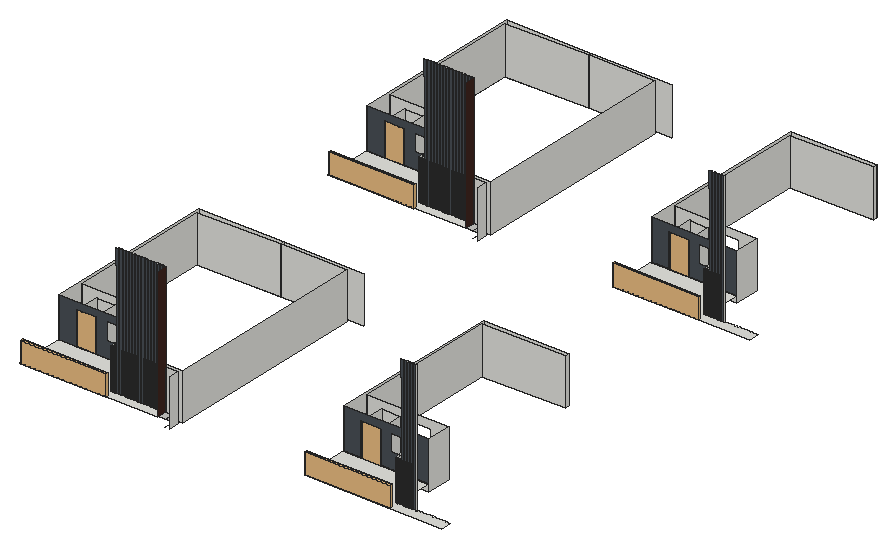
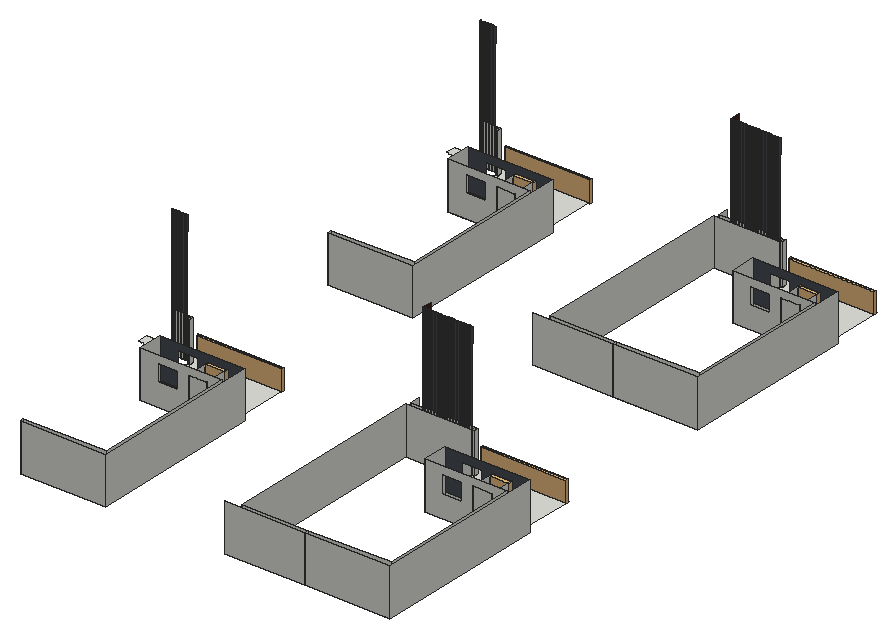
# SketchUp Ruby script. Lengths in inches.
U = 1.inch
M = Sketchup.active_model
def pt(a) = Geom::Point3d.new(a.map { |v| v * U })
def face(e, loops, mat)
  f = e.add_face(loops[0].map { |a| pt(a) })
  loops[1..].each { |l| e.add_face(l.map { |a| pt(a) }).erase! }
  f.material = f.back_material = mat if mat
  f
end
# faces: each face lists its corners as indices into pts; further lists are holes
def faces(e, pts, list, mat = nil) = list.each { |f| face(e, (f[0].is_a?(Array) ? f : [f]).map { |l| l.map { |i| pts[i] } }, mat) }
# xy, xz, yz: faces in a plane at the given z, y or x. An outline is a flat list of corners, or four numbers for a rectangle; further outlines are holes
def ring(l) = l.size == 4 ? [[l[0], l[1]], [l[2], l[1]], [l[2], l[3]], [l[0], l[3]]] : l.each_slice(2).to_a
def flat(e, list, mat, &to3) = list.each { |f| face(e, (f[0].is_a?(Array) ? f : [f]).map { |l| ring(l).map { |u, v| to3.(u, v) } }, mat) }
def xy(e, z, list, mat = nil) = flat(e, list, mat) { |x, y| [x, y, z] }
def xz(e, y, list, mat = nil) = flat(e, list, mat) { |x, z| [x, y, z] }
def yz(e, x, list, mat = nil) = flat(e, list, mat) { |y, z| [x, y, z] }
def lines(e, pts, list) = list.each { |a, b| e.add_line(pt(pts[a]), pt(pts[b])) }
# prism: a flat outline (further loops are holes) pulled along v
def prism(e, loops, v, mat = nil)
  f = face(e, loops, mat); d = Geom::Vector3d.new(v.map { |x| x * U })
  f.pushpull(f.normal.samedirection?(d) ? d.length : -d.length)
end
def box(e, o, s, mat = nil) = prism(e, [[o, [o[0] + s[0], o[1], o[2]], [o[0] + s[0], o[1] + s[1], o[2]], [o[0], o[1] + s[1], o[2]]]], [0, 0, s[2]], mat)
def at(x, y, z, deg = 0) = Geom::Transformation.translation(pt([x, y, z])) * Geom::Transformation.rotation(ORIGIN, Z_AXIS, deg.degrees)
def axes(o, x, y, z) = Geom::Transformation.new([*x, 0, *y, 0, *z, 0, *pt(o).to_a, 1])
def part(name) = M.definitions.add(name)
# library, detail: a bought-in or finely detailed component or shape, given as its bounding box
def library(name, o, s) = part(name).tap { |d| box(d.entities, o, s) }
def detail(e, o, s) = box(e.add_group.entities, o, s)
def put(e, d, t, mat = nil) = e.add_instance(d, t).tap { |i| i.material = mat if mat }
def group(e, t, mat = nil) = e.add_group.tap { |g| g.transformation = t; g.material = mat if mat }.entities
root = M.entities
M.materials.add("[0043_SaddleBrown]").color = [63, 38, 31]
M.materials.add("[Formica Blue]").color = [73, 80, 86]
c1 = library("door (1)",[38.93,25.48,0],[40,9.94,82.68])
c2 = library("Glass Railing",[0,0,0],[139.5,4.76,42])
xy(root,384.25,[[348.1875,438.72,353.97,447.84],[1072.625,438.72,1078.41,447.84],[137.5,535.375,137.5,980.35,353.97,980.35,353.97,971.23,144.84,965.96,144.84,540.48,353.97,540.48,353.97,535.375],[861.9375,535.375,861.9375,980.35,1078.41,980.35,1078.41,971.23,869.28,965.96,869.28,540.48,1078.41,540.48,1078.41,535.375],[144.84,540.48,353.97,598.8125],
  [869.28,540.48,1078.41,598.8125],[348.1875,1419.07,353.97,1428.19],[1072.625,1419.07,1078.41,1428.19],[137.5,1515.73,137.5,1960.7,353.97,1960.7,353.97,1951.58,144.84,1946.3125,144.84,1520.83,353.97,1520.83,353.97,1515.73],[861.9375,1515.73,861.9375,1960.7,1078.41,1960.7,1078.41,1951.58,869.28,1946.3125,869.28,1520.83,1078.41,1520.83,1078.41,1515.73],
  [144.84,1520.83,353.97,1579.16],[869.28,1520.83,1078.41,1579.16]])
xy(root,401.6875,[[137.5,412.04,487.0625,412.04,487.0625,437.1,481.3,437.1,481.3,438.72,479.0625,438.72,479.0625,437.1,473.3,437.1,473.3,438.72,471.0625,438.72,471.0625,437.1,465.3,437.1,465.3,438.72,463.0625,438.72,463.0625,437.1,457.3,437.1,457.3,438.72,455.0625,438.72,455.0625,437.1,449.3,437.1,449.3,438.72,447.0625,438.72,447.0625,437.1,441.3,437.1,441.3,438.72,439.0625,438.72,439.0625,437.1,433.3,437.1,433.3,438.72,431.0625,438.72,431.0625,437.1,425.3,437.1,425.3,438.72,423.0625,438.72,423.0625,437.1,417.3,437.1,417.3,438.72,415.0625,438.72,415.0625,437.1,409.3,437.1,409.3,438.72,407.0625,438.72,407.0625,437.1,401.3,437.1,401.3,438.72,399.0625,438.72,399.0625,437.1,393.3,437.1,393.3,438.72,391.0625,438.72,391.0625,437.1,385.3,437.1,385.3,438.72,383.0625,438.72,383.0625,437.1,377.3,437.1,377.3,438.72,375.0625,438.72,375.0625,437.1,369.3,437.1,369.3,438.72,367.0625,438.72,367.0625,437.1,361.3,437.1,361.3,438.72,358.875,438.72,358.875,437.1,353.97,437.1,353.97,438.72,352.41,438.72,352.41,437.1,348.1875,437.1,348.1875,447.84,353.97,447.84,353.97,535.375,137.5,535.375],[861.9375,412.04,1211.5,412.04,1211.5,437.1,1205.74,437.1,1205.74,438.72,1203.5,438.72,1203.5,437.1,1197.74,437.1,1197.74,438.72,1195.5,438.72,1195.5,437.1,1189.74,437.1,1189.74,438.72,1187.5,438.72,1187.5,437.1,1181.74,437.1,1181.74,438.72,1179.5,438.72,1179.5,437.1,1173.74,437.1,1173.74,438.72,1171.5,438.72,1171.5,437.1,1165.74,437.1,1165.74,438.72,1163.5,438.72,1163.5,437.1,1157.74,437.1,1157.74,438.72,1155.5,438.72,1155.5,437.1,1149.74,437.1,1149.74,438.72,1147.5,438.72,1147.5,437.1,1141.74,437.1,1141.74,438.72,1139.5,438.72,1139.5,437.1,1133.74,437.1,1133.74,438.72,1131.5,438.72,1131.5,437.1,1125.74,437.1,1125.74,438.72,1123.5,438.72,1123.5,437.1,1117.74,437.1,1117.74,438.72,1115.5,438.72,1115.5,437.1,1109.74,437.1,1109.74,438.72,1107.5,438.72,1107.5,437.1,1101.74,437.1,1101.74,438.72,1099.5,438.72,1099.5,437.1,1093.74,437.1,1093.74,438.72,1091.5,438.72,1091.5,437.1,1085.74,437.1,1085.74,438.72,1083.3125,438.72,1083.3125,437.1,1078.41,437.1,1078.41,438.72,1076.85,438.72,1076.85,437.1,1072.625,437.1,1072.625,447.84,1078.41,447.84,1078.41,535.375,861.9375,535.375],[348.1875,437.1,352.41,438.72],[353.97,437.1,358.875,438.72],[361.3,437.1,367.0625,438.72],
  [369.3,437.1,375.0625,438.72],[377.3,437.1,383.0625,438.72],[385.3,437.1,391.0625,438.72],[393.3,437.1,399.0625,438.72],[401.3,437.1,407.0625,438.72],
  [409.3,437.1,415.0625,438.72],[417.3,437.1,423.0625,438.72],[425.3,437.1,431.0625,438.72],[433.3,437.1,439.0625,438.72],[441.3,437.1,447.0625,438.72],
  [449.3,437.1,455.0625,438.72],[457.3,437.1,463.0625,438.72],[465.3,437.1,471.0625,438.72],[473.3,437.1,479.0625,438.72],[481.3,437.1,487.0625,438.72],
  [1072.625,437.1,1076.85,438.72],[1078.41,437.1,1083.3125,438.72],[1085.74,437.1,1091.5,438.72],[1093.74,437.1,1099.5,438.72],[1101.74,437.1,1107.5,438.72],
  [1109.74,437.1,1115.5,438.72],[1117.74,437.1,1123.5,438.72],[1125.74,437.1,1131.5,438.72],[183.3,535.375,231.3,598.8125],[907.74,535.375,955.74,598.8125],
  [137.5,1392.39,487.0625,1392.39,487.0625,1417.45,481.3,1417.45,481.3,1419.07,479.0625,1419.07,479.0625,1417.45,473.3,1417.45,473.3,1419.07,471.0625,1419.07,471.0625,1417.45,465.3,1417.45,465.3,1419.07,463.0625,1419.07,463.0625,1417.45,457.3,1417.45,457.3,1419.07,455.0625,1419.07,455.0625,1417.45,449.3,1417.45,449.3,1419.07,447.0625,1419.07,447.0625,1417.45,441.3,1417.45,441.3,1419.07,439.0625,1419.07,439.0625,1417.45,433.3,1417.45,433.3,1419.07,431.0625,1419.07,431.0625,1417.45,425.3,1417.45,425.3,1419.07,423.0625,1419.07,423.0625,1417.45,417.3,1417.45,417.3,1419.07,415.0625,1419.07,415.0625,1417.45,409.3,1417.45,409.3,1419.07,407.0625,1419.07,407.0625,1417.45,401.3,1417.45,401.3,1419.07,399.0625,1419.07,399.0625,1417.45,393.3,1417.45,393.3,1419.07,391.0625,1419.07,391.0625,1417.45,385.3,1417.45,385.3,1419.07,383.0625,1419.07,383.0625,1417.45,377.3,1417.45,377.3,1419.07,375.0625,1419.07,375.0625,1417.45,369.3,1417.45,369.3,1419.07,367.0625,1419.07,367.0625,1417.45,361.3,1417.45,361.3,1419.07,358.875,1419.07,358.875,1417.45,353.97,1417.45,353.97,1419.07,352.41,1419.07,352.41,1417.45,348.1875,1417.45,348.1875,1428.19,353.97,1428.19,353.97,1515.73,137.5,1515.73],[861.9375,1392.39,1211.5,1392.39,1211.5,1417.45,1205.74,1417.45,1205.74,1419.07,1203.5,1419.07,1203.5,1417.45,1197.74,1417.45,1197.74,1419.07,1195.5,1419.07,1195.5,1417.45,1189.74,1417.45,1189.74,1419.07,1187.5,1419.07,1187.5,1417.45,1181.74,1417.45,1181.74,1419.07,1179.5,1419.07,1179.5,1417.45,1173.74,1417.45,1173.74,1419.07,1171.5,1419.07,1171.5,1417.45,1165.74,1417.45,1165.74,1419.07,1163.5,1419.07,1163.5,1417.45,1157.74,1417.45,1157.74,1419.07,1155.5,1419.07,1155.5,1417.45,1149.74,1417.45,1149.74,1419.07,1147.5,1419.07,1147.5,1417.45,1141.74,1417.45,1141.74,1419.07,1139.5,1419.07,1139.5,1417.45,1133.74,1417.45,1133.74,1419.07,1131.5,1419.07,1131.5,1417.45,1125.74,1417.45,1125.74,1419.07,1123.5,1419.07,1123.5,1417.45,1117.74,1417.45,1117.74,1419.07,1115.5,1419.07,1115.5,1417.45,1109.74,1417.45,1109.74,1419.07,1107.5,1419.07,1107.5,1417.45,1101.74,1417.45,1101.74,1419.07,1099.5,1419.07,1099.5,1417.45,1093.74,1417.45,1093.74,1419.07,1091.5,1419.07,1091.5,1417.45,1085.74,1417.45,1085.74,1419.07,1083.3125,1419.07,1083.3125,1417.45,1078.41,1417.45,1078.41,1419.07,1076.85,1419.07,1076.85,1417.45,1072.625,1417.45,1072.625,1428.19,1078.41,1428.19,1078.41,1515.73,861.9375,1515.73],[348.1875,1417.45,352.41,1419.07],[353.97,1417.45,358.875,1419.07],[361.3,1417.45,367.0625,1419.07],
  [369.3,1417.45,375.0625,1419.07],[377.3,1417.45,383.0625,1419.07],[385.3,1417.45,391.0625,1419.07],[393.3,1417.45,399.0625,1419.07],[401.3,1417.45,407.0625,1419.07],
  [409.3,1417.45,415.0625,1419.07],[417.3,1417.45,423.0625,1419.07],[425.3,1417.45,431.0625,1419.07],[433.3,1417.45,439.0625,1419.07],[441.3,1417.45,447.0625,1419.07],
  [449.3,1417.45,455.0625,1419.07],[457.3,1417.45,463.0625,1419.07],[465.3,1417.45,471.0625,1419.07],[473.3,1417.45,479.0625,1419.07],[481.3,1417.45,487.0625,1419.07],
  [1072.625,1417.45,1076.85,1419.07],[1078.41,1417.45,1083.3125,1419.07],[1085.74,1417.45,1091.5,1419.07],[1093.74,1417.45,1099.5,1419.07],[1101.74,1417.45,1107.5,1419.07],
  [1109.74,1417.45,1115.5,1419.07],[1117.74,1417.45,1123.5,1419.07],[183.3,1515.73,231.3,1579.16],[907.74,1515.73,955.74,1579.16]])
xz(root,437.1,[[348.1875,401.6875,352.41,504.25],[353.97,401.6875,358.875,504.25],[361.3,401.6875,367.0625,401.6875,367.0625,733.125,361.3,733.125,361.3,693.65,363.73,693.65,363.73,504.25,361.3,504.25],[369.3,401.6875,375.0625,733.125],[377.3,401.6875,383.0625,733.125],
  [385.3,401.6875,391.0625,733.125],[393.3,401.6875,399.0625,733.125],[401.3,401.6875,407.0625,733.125],[409.3,401.6875,415.0625,733.125],[417.3,401.6875,423.0625,733.125],
  [425.3,401.6875,431.0625,733.125],[433.3,401.6875,439.0625,733.125],[441.3,401.6875,447.0625,733.125],[449.3,401.6875,455.0625,733.125],[457.3,401.6875,463.0625,733.125],
  [465.3,401.6875,471.0625,733.125],[473.3,401.6875,479.0625,733.125],[481.3,401.6875,487.0625,733.125],[1072.625,401.6875,1076.85,504.25],[1078.41,401.6875,1083.3125,504.25],
  [1085.74,401.6875,1091.5,401.6875,1091.5,733.125,1085.74,733.125,1085.74,693.65,1088.17,693.65,1088.17,504.25,1085.74,504.25],[1093.74,401.6875,1099.5,733.125],[1101.74,401.6875,1107.5,733.125],[1109.74,401.6875,1115.5,733.125],[1117.74,401.6875,1123.5,733.125]],"[Formica Blue]")
xz(root,438.72,[[348.1875,384.25,353.97,401.6875],[353.97,384.25,504.5,401.6875],[1072.625,384.25,1078.41,401.6875]])
xz(root,438.72,[[352.41,401.6875,353.97,504.25],[358.875,401.6875,361.3,504.25],[367.0625,401.6875,369.3,733.125],[375.0625,401.6875,377.3,733.125],[383.0625,401.6875,385.3,733.125],
  [391.0625,401.6875,393.3,733.125],[399.0625,401.6875,401.3,733.125],[407.0625,401.6875,409.3,733.125],[415.0625,401.6875,417.3,733.125],[423.0625,401.6875,425.3,733.125],
  [431.0625,401.6875,433.3,733.125],[439.0625,401.6875,441.3,733.125],[447.0625,401.6875,449.3,733.125],[455.0625,401.6875,457.3,733.125],[463.0625,401.6875,465.3,733.125],
  [471.0625,401.6875,473.3,733.125],[479.0625,401.6875,481.3,733.125],[1076.85,401.6875,1078.41,504.25],[1083.3125,401.6875,1085.74,504.25],[1091.5,401.6875,1093.74,733.125],
  [1099.5,401.6875,1101.74,733.125],[1107.5,401.6875,1109.74,733.125],[1115.5,401.6875,1117.74,733.125],[1123.5,401.6875,1125.74,733.125]],"[Formica Blue]")
xz(root,447.84,[[348.1875,384.25,353.97,401.6875],[353.97,384.25,521.63,504.25],[1072.625,384.25,1078.41,401.6875],[348.1875,401.6875,353.97,504.25],[1072.625,401.6875,1078.41,504.25]])
xz(root,535.375,[[137.5,384.25,353.97,401.6875],[861.9375,384.25,1078.41,401.6875]])
xz(root,535.375,[[[137.5,401.6875,183.3,401.6875,183.3,485.6875,231.3,485.6875,231.3,401.6875,353.97,401.6875,353.97,504.25,137.5,504.25],[258.09,441.5,309.84,485.6875]],[[861.9375,401.6875,907.74,401.6875,907.74,485.6875,955.74,485.6875,955.74,401.6875,1078.41,401.6875,1078.41,504.25,861.9375,504.25],[982.53,441.5,1034.28,485.6875]]],"[Formica Blue]")
xz(root,598.8125,[[[144.84,384.25,353.97,504.25],[183.3,401.6875,231.3,485.6875],[258.09,441.5,309.84,485.6875]],[[869.28,384.25,1078.41,504.25],[907.74,401.6875,955.74,485.6875],[982.53,441.5,1034.28,485.6875]],[183.3,401.6875,231.3,485.6875],[907.74,401.6875,955.74,485.6875]])
xz(root,971.23,[[353.97,384.25,521.63,504.25]])
xz(root,980.35,[[137.5,384.25,353.97,504.25],[353.97,384.25,558.625,504.25],[861.9375,384.25,1078.41,504.25]])
xz(root,1417.45,[[348.1875,401.6875,352.41,504.25],[353.97,401.6875,358.875,504.25],[361.3,401.6875,367.0625,401.6875,367.0625,733.125,361.3,733.125,361.3,693.65,363.73,693.65,363.73,504.25,361.3,504.25],[369.3,401.6875,375.0625,733.125],[377.3,401.6875,383.0625,733.125],
  [385.3,401.6875,391.0625,733.125],[393.3,401.6875,399.0625,733.125],[401.3,401.6875,407.0625,733.125],[409.3,401.6875,415.0625,733.125],[417.3,401.6875,423.0625,733.125],
  [425.3,401.6875,431.0625,733.125],[433.3,401.6875,439.0625,733.125],[441.3,401.6875,447.0625,733.125],[449.3,401.6875,455.0625,733.125],[457.3,401.6875,463.0625,733.125],
  [465.3,401.6875,471.0625,733.125],[473.3,401.6875,479.0625,733.125],[481.3,401.6875,487.0625,733.125],[1072.625,401.6875,1076.85,504.25],[1078.41,401.6875,1083.3125,504.25],
  [1085.74,401.6875,1091.5,401.6875,1091.5,733.125,1085.74,733.125,1085.74,693.65,1088.17,693.65,1088.17,504.25,1085.74,504.25],[1093.74,401.6875,1099.5,733.125],[1101.74,401.6875,1107.5,733.125],[1109.74,401.6875,1115.5,733.125],[1117.74,401.6875,1123.5,733.125]],"[Formica Blue]")
xz(root,1419.07,[[348.1875,384.25,353.97,401.6875],[353.97,384.25,504.5,401.6875],[1072.625,384.25,1078.41,401.6875]])
xz(root,1419.07,[[352.41,401.6875,353.97,504.25],[358.875,401.6875,361.3,504.25],[367.0625,401.6875,369.3,733.125],[375.0625,401.6875,377.3,733.125],[383.0625,401.6875,385.3,733.125],
  [391.0625,401.6875,393.3,733.125],[399.0625,401.6875,401.3,733.125],[407.0625,401.6875,409.3,733.125],[415.0625,401.6875,417.3,733.125],[423.0625,401.6875,425.3,733.125],
  [431.0625,401.6875,433.3,733.125],[439.0625,401.6875,441.3,733.125],[447.0625,401.6875,449.3,733.125],[455.0625,401.6875,457.3,733.125],[463.0625,401.6875,465.3,733.125],
  [471.0625,401.6875,473.3,733.125],[479.0625,401.6875,481.3,733.125],[1076.85,401.6875,1078.41,504.25],[1083.3125,401.6875,1085.74,504.25],[1091.5,401.6875,1093.74,733.125],
  [1099.5,401.6875,1101.74,733.125],[1107.5,401.6875,1109.74,733.125],[1115.5,401.6875,1117.74,733.125],[1123.5,401.6875,1125.74,733.125]],"[Formica Blue]")
xz(root,1428.19,[[348.1875,384.25,353.97,401.6875],[353.97,384.25,521.63,504.25],[1072.625,384.25,1078.41,401.6875],[348.1875,401.6875,353.97,504.25],[1072.625,401.6875,1078.41,504.25]])
xz(root,1515.73,[[137.5,384.25,353.97,401.6875],[861.9375,384.25,1078.41,401.6875]])
xz(root,1515.73,[[[137.5,401.6875,183.3,401.6875,183.3,485.6875,231.3,485.6875,231.3,401.6875,353.97,401.6875,353.97,504.25,137.5,504.25],[258.09,441.5,309.84,485.6875]],[[861.9375,401.6875,907.74,401.6875,907.74,485.6875,955.74,485.6875,955.74,401.6875,1078.41,401.6875,1078.41,504.25,861.9375,504.25],[982.53,441.5,1034.28,485.6875]]],"[Formica Blue]")
xz(root,1579.16,[[[144.84,384.25,353.97,504.25],[183.3,401.6875,231.3,485.6875],[258.09,441.5,309.84,485.6875]],[[869.28,384.25,1078.41,504.25],[907.74,401.6875,955.74,485.6875],[982.53,441.5,1034.28,485.6875]],[183.3,401.6875,231.3,485.6875],[907.74,401.6875,955.74,485.6875]])
xz(root,1951.58,[[353.97,384.25,521.63,504.25]])
xz(root,1960.7,[[137.5,384.25,353.97,504.25],[353.97,384.25,558.625,504.25],[861.9375,384.25,1078.41,504.25]])
yz(root,137.5,[[535.375,384.25,980.35,504.25],[1515.73,384.25,1960.7,504.25]])
yz(root,144.84,[[598.8125,384.25,965.96,504.25],[1579.16,384.25,1946.3125,504.25]])
yz(root,183.3,[[535.375,401.6875,598.8125,485.6875],[1515.73,401.6875,1579.16,485.6875]])
yz(root,231.3,[[535.375,401.6875,598.8125,485.6875],[1515.73,401.6875,1579.16,485.6875]])
yz(root,348.1875,[[438.72,384.25,447.84,401.6875],[1419.07,384.25,1428.19,401.6875],[437.1,401.6875,447.84,504.25],[1417.45,401.6875,1428.19,504.25]])
yz(root,352.41,[[437.1,401.6875,438.72,504.25],[1417.45,401.6875,1419.07,504.25]])
yz(root,353.97,[[438.72,384.25,447.84,504.25],[535.375,384.25,598.8125,504.25],[971.23,384.25,980.35,504.25],[1419.07,384.25,1428.19,504.25],[1515.73,384.25,1579.16,504.25],
  [1951.58,384.25,1960.7,504.25],[437.1,401.6875,438.72,504.25],[1417.45,401.6875,1419.07,504.25]])
yz(root,358.875,[[437.1,401.6875,438.72,504.25],[1417.45,401.6875,1419.07,504.25]])
yz(root,361.3,[[437.1,401.6875,438.72,504.25],[1417.45,401.6875,1419.07,504.25]])
yz(root,367.0625,[[437.1,401.6875,438.72,504.25],[1417.45,401.6875,1419.07,504.25]])
yz(root,369.3,[[437.1,401.6875,438.72,733.125],[1417.45,401.6875,1419.07,733.125]])
yz(root,375.0625,[[437.1,401.6875,438.72,504.25],[1417.45,401.6875,1419.07,504.25]])
yz(root,377.3,[[437.1,401.6875,438.72,733.125],[1417.45,401.6875,1419.07,733.125]])
yz(root,383.0625,[[437.1,401.6875,438.72,504.25],[1417.45,401.6875,1419.07,504.25]])
yz(root,385.3,[[437.1,401.6875,438.72,733.125],[1417.45,401.6875,1419.07,733.125]])
yz(root,391.0625,[[437.1,401.6875,438.72,504.25],[1417.45,401.6875,1419.07,504.25]])
yz(root,393.3,[[437.1,401.6875,438.72,733.125],[1417.45,401.6875,1419.07,733.125]])
yz(root,399.0625,[[437.1,401.6875,438.72,504.25],[1417.45,401.6875,1419.07,504.25]])
yz(root,401.3,[[437.1,401.6875,438.72,733.125],[1417.45,401.6875,1419.07,733.125]])
yz(root,407.0625,[[437.1,401.6875,438.72,504.25],[1417.45,401.6875,1419.07,504.25]])
yz(root,409.3,[[437.1,401.6875,438.72,733.125],[1417.45,401.6875,1419.07,733.125]])
yz(root,415.0625,[[437.1,401.6875,438.72,504.25],[1417.45,401.6875,1419.07,504.25]])
yz(root,417.3,[[437.1,401.6875,438.72,733.125],[1417.45,401.6875,1419.07,733.125]])
yz(root,423.0625,[[437.1,401.6875,438.72,504.25],[1417.45,401.6875,1419.07,504.25]])
yz(root,425.3,[[437.1,401.6875,438.72,733.125],[1417.45,401.6875,1419.07,733.125]])
yz(root,431.0625,[[437.1,401.6875,438.72,504.25],[1417.45,401.6875,1419.07,504.25]])
yz(root,433.3,[[437.1,401.6875,438.72,733.125],[1417.45,401.6875,1419.07,733.125]])
yz(root,439.0625,[[437.1,401.6875,438.72,504.25],[1417.45,401.6875,1419.07,504.25]])
yz(root,441.3,[[437.1,401.6875,438.72,733.125],[1417.45,401.6875,1419.07,733.125]])
yz(root,447.0625,[[437.1,401.6875,438.72,504.25],[1417.45,401.6875,1419.07,504.25]])
yz(root,449.3,[[437.1,401.6875,438.72,733.125],[1417.45,401.6875,1419.07,733.125]])
yz(root,455.0625,[[437.1,401.6875,438.72,504.25],[1417.45,401.6875,1419.07,504.25]])
yz(root,457.3,[[437.1,401.6875,438.72,733.125],[1417.45,401.6875,1419.07,733.125]])
yz(root,463.0625,[[437.1,401.6875,438.72,504.25],[1417.45,401.6875,1419.07,504.25]])
yz(root,465.3,[[437.1,401.6875,438.72,733.125],[1417.45,401.6875,1419.07,733.125]])
yz(root,471.0625,[[437.1,401.6875,438.72,504.25],[1417.45,401.6875,1419.07,504.25]])
yz(root,473.3,[[437.1,401.6875,438.72,733.125],[1417.45,401.6875,1419.07,733.125]])
yz(root,479.0625,[[437.1,401.6875,438.72,504.25],[1417.45,401.6875,1419.07,504.25]])
yz(root,481.3,[[437.1,401.6875,438.72,733.125],[1417.45,401.6875,1419.07,733.125]])
yz(root,487.0625,[[437.1,401.6875,438.72,504.25],[1417.45,401.6875,1419.07,504.25]])
yz(root,487.0625,[[412.04,401.6875,437.1,733.125],[1392.39,401.6875,1417.45,733.125]],"[0043_SaddleBrown]")
yz(root,517.3125,[[412.04,384.25,438.72,384.25,438.73,409.48,438.72,412.48,438.72,504.25,412.04,504.25],[1392.39,384.25,1419.07,384.25,1419.08,409.48,1419.07,412.48,1419.07,504.25,1392.39,504.25]])
yz(root,521.63,[[447.84,384.25,971.23,504.25],[1428.19,384.25,1951.58,504.25]])
yz(root,861.9375,[[535.375,384.25,980.35,504.25],[1515.73,384.25,1960.7,504.25]])
yz(root,869.28,[[598.8125,384.25,965.96,504.25],[1579.16,384.25,1946.3125,504.25]])
yz(root,907.74,[[535.375,401.6875,598.8125,485.6875],[1515.73,401.6875,1579.16,485.6875]])
yz(root,955.74,[[535.375,401.6875,598.8125,485.6875],[1515.73,401.6875,1579.16,485.6875]])
yz(root,1072.625,[[438.72,384.25,447.84,401.6875],[1419.07,384.25,1428.19,401.6875],[437.1,401.6875,447.84,504.25],[1417.45,401.6875,1428.19,504.25]])
yz(root,1076.85,[[437.1,401.6875,438.72,504.25],[1417.45,401.6875,1419.07,504.25]])
yz(root,1078.41,[[438.72,384.25,447.84,504.25],[535.375,384.25,598.8125,504.25],[971.23,384.25,980.35,504.25],[1419.07,384.25,1428.19,504.25],[1515.73,384.25,1579.16,504.25],
  [1951.58,384.25,1960.7,504.25],[437.1,401.6875,438.72,504.25],[1417.45,401.6875,1419.07,504.25]])
yz(root,1083.3125,[[437.1,401.6875,438.72,504.25],[1417.45,401.6875,1419.07,504.25]])
yz(root,1085.74,[[437.1,401.6875,438.72,504.25],[1417.45,401.6875,1419.07,504.25]])
yz(root,1091.5,[[437.1,401.6875,438.72,504.25],[1417.45,401.6875,1419.07,504.25]])
yz(root,1093.74,[[437.1,401.6875,438.72,733.125],[1417.45,401.6875,1419.07,733.125]])
yz(root,1099.5,[[437.1,401.6875,438.72,504.25],[1417.45,401.6875,1419.07,504.25]])
yz(root,1101.74,[[437.1,401.6875,438.72,733.125],[1417.45,401.6875,1419.07,733.125]])
yz(root,1107.5,[[437.1,401.6875,438.72,504.25],[1417.45,401.6875,1419.07,504.25]])
yz(root,1109.74,[[437.1,401.6875,438.72,733.125],[1417.45,401.6875,1419.07,733.125]])
yz(root,1115.5,[[437.1,401.6875,438.72,504.25],[1417.45,401.6875,1419.07,504.25]])
yz(root,1117.74,[[437.1,401.6875,438.72,733.125],[1417.45,401.6875,1419.07,733.125]])
yz(root,1123.5,[[437.1,401.6875,438.72,504.25],[1417.45,401.6875,1419.07,504.25]])
yz(root,1125.74,[[437.1,401.6875,438.72,733.125],[1417.45,401.6875,1419.07,733.125]])
p = [[504.5,438.72,384.25],[517.3125,438.72,384.25],[517.3125,438.73,409.48],[517.3125,438.72,412.48],[517.3125,438.72,504.25],[487.0625,438.72,504.25],
  [487.0625,438.72,401.6875],[504.5,438.72,401.6875],[144.84,965.96,384.25],[353.97,971.23,384.25],[353.97,971.23,504.25],[144.84,965.96,504.25],
  [869.28,965.96,384.25],[1078.41,971.23,384.25],[1078.41,971.23,504.25],[869.28,965.96,504.25],[504.5,1419.07,384.25],[517.3125,1419.07,384.25],
  [517.3125,1419.08,409.48],[517.3125,1419.07,412.48],[517.3125,1419.07,504.25],[487.0625,1419.07,504.25],[487.0625,1419.07,401.6875],[504.5,1419.07,401.6875],
  [144.84,1946.3125,384.25],[353.97,1951.58,384.25],[353.97,1951.58,504.25],[144.84,1946.3125,504.25],[869.28,1946.3125,384.25],[1078.41,1951.58,384.25],
  [1078.41,1951.58,504.25],[869.28,1946.3125,504.25],[504.5,412.04,401.6875],[504.5,412.04,384.25],[504.5,1392.39,401.6875],[504.5,1392.39,384.25]]
faces(root,p,[[0,1,2,3,4,5,6,7],[8,9,10,11],[12,13,14,15],[16,17,18,19,20,21,22,23],[24,25,26,27],[28,29,30,31]])
lines(root,p,[[7,32],[0,33],[23,34],[16,35]])
put(root,c1,axes([133.81,509.89,401.6875],[1.2351,0,0],[0,1,0],[0,0,1.016]))
put(root,c1,axes([133.81,1490.24,401.6875],[1.2351,0,0],[0,1,0],[0,0,1.016]))
put(root,c2,axes([137.5,413.41,399.63],[1.55466,0,0],[0,1.27,0],[0,0,1.27]))
put(root,c2,axes([137.5,1393.76,399.63],[1.55466,0,0],[0,1.27,0],[0,0,1.27]))
put(root,c1,axes([858.25,509.89,401.6875],[1.2351,0,0],[0,1,0],[0,0,1.016]))
put(root,c1,axes([858.25,1490.24,401.6875],[1.2351,0,0],[0,1,0],[0,0,1.016]))
put(root,c2,axes([861.9375,413.41,399.63],[1.55466,0,0],[0,1.27,0],[0,0,1.27]))
put(root,c2,axes([861.9375,1393.76,399.63],[1.55466,0,0],[0,1.27,0],[0,0,1.27]))
